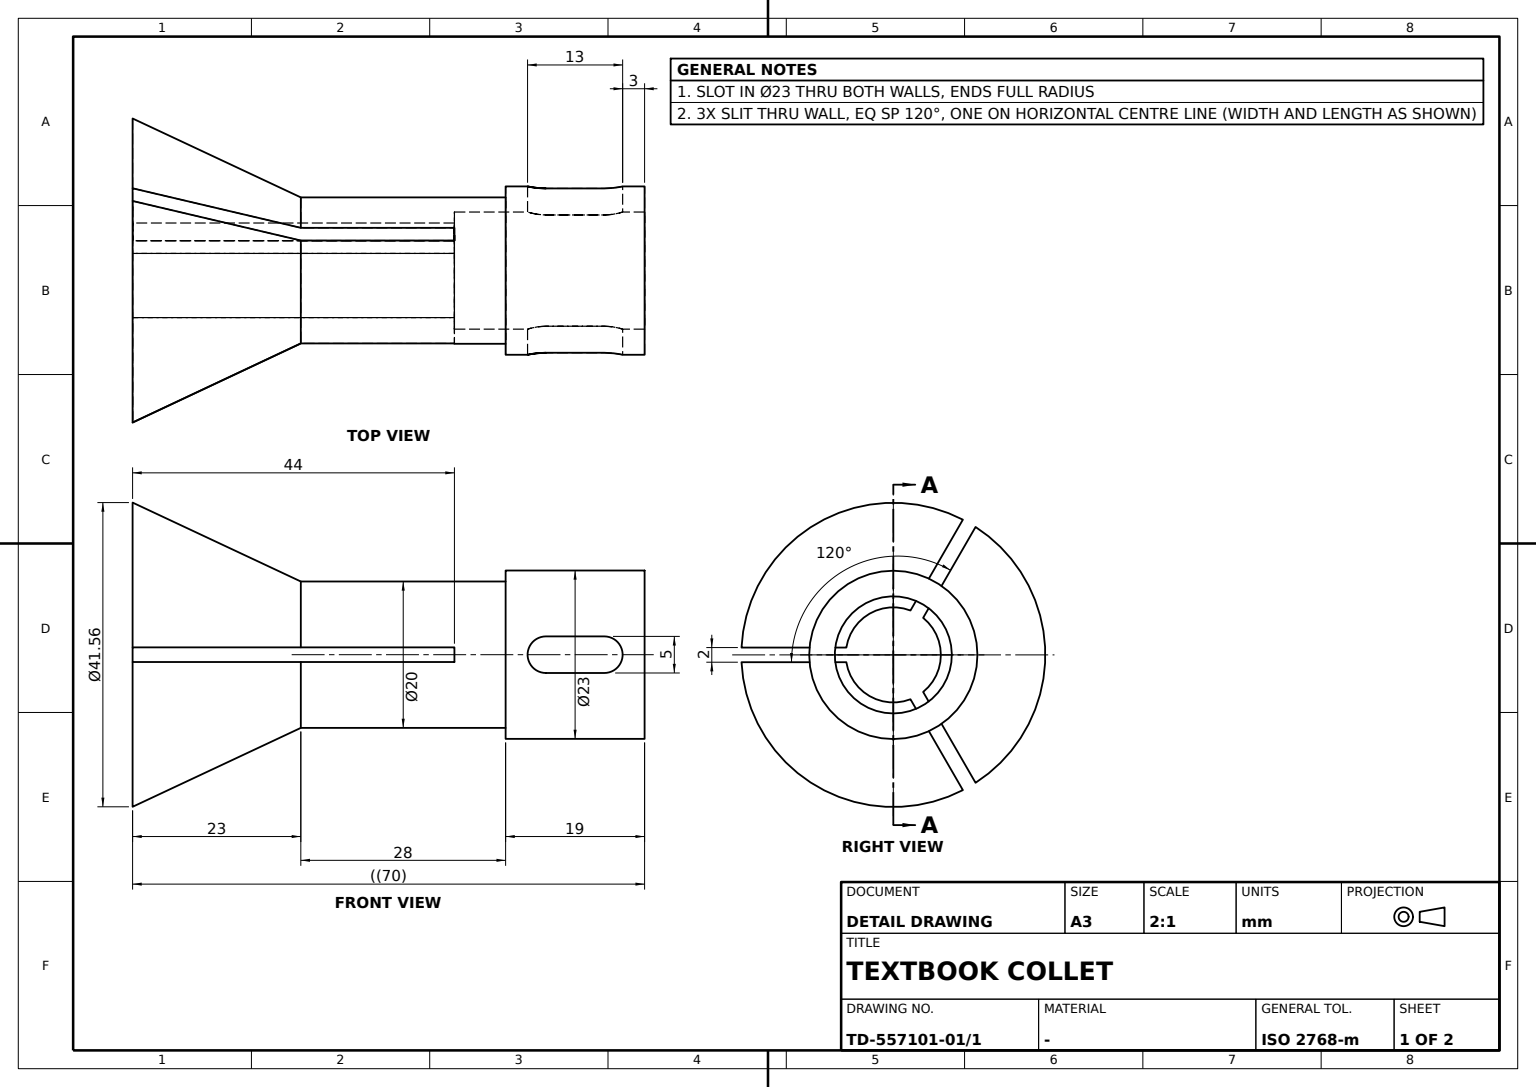
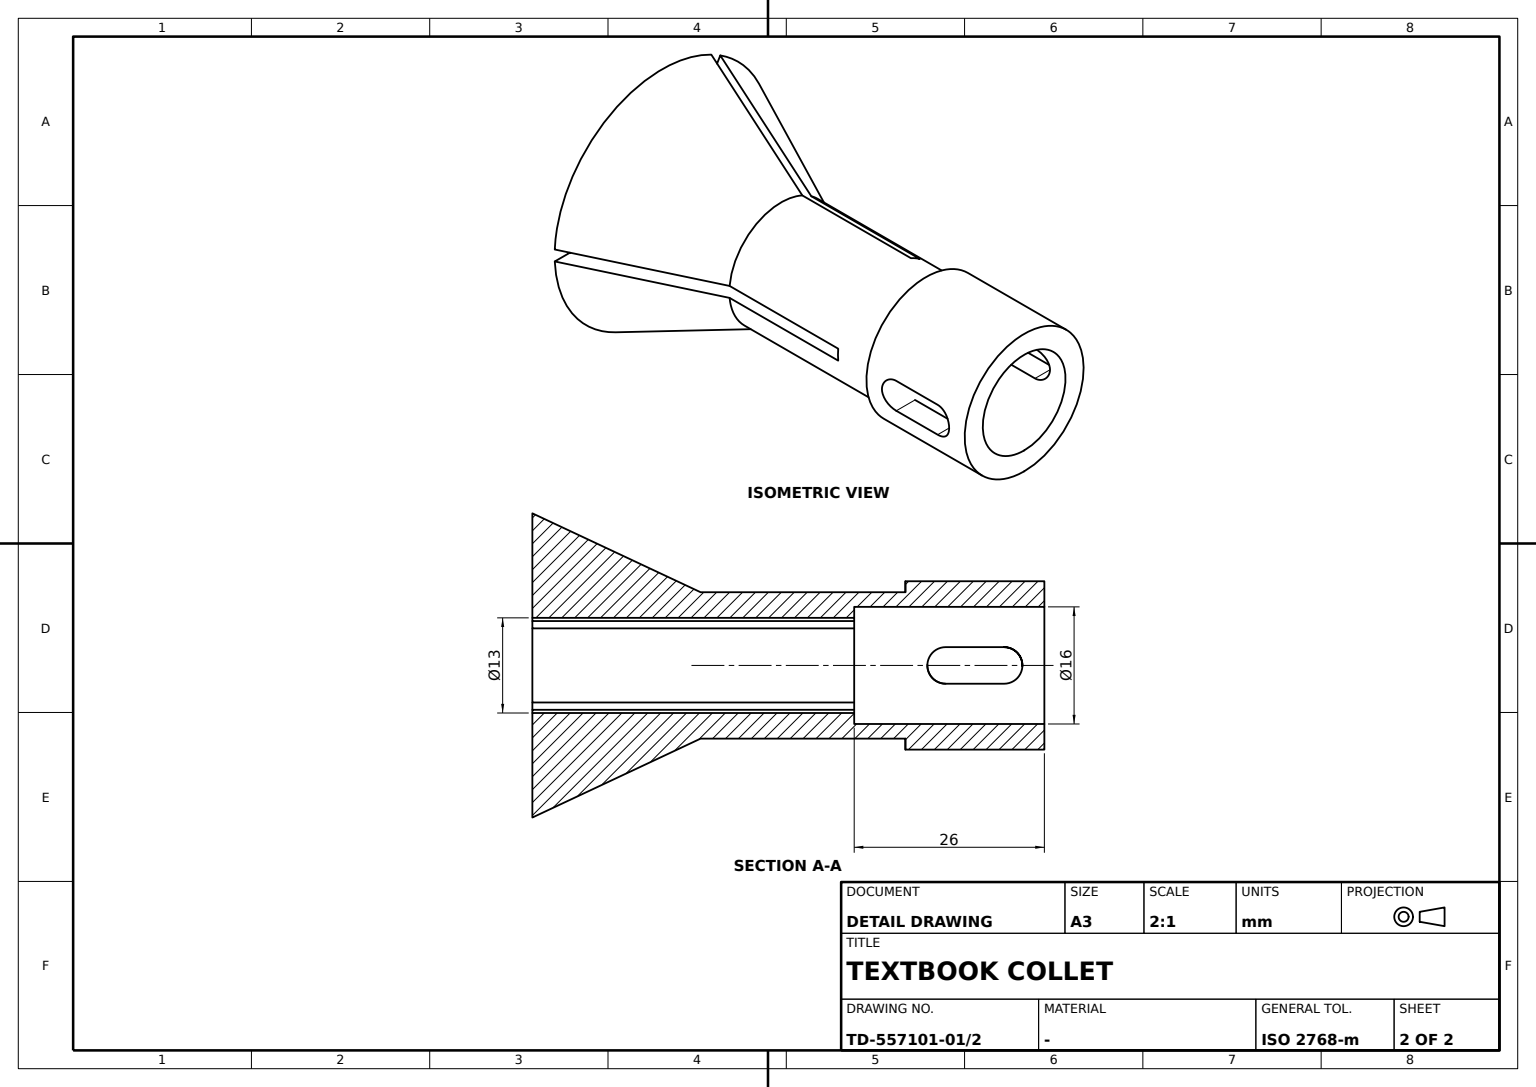
ISO-10303-21;
HEADER;
FILE_DESCRIPTION((''),'2;1');
FILE_NAME('','',(''),(''),'','','');
FILE_SCHEMA(('AUTOMOTIVE_DESIGN'));
ENDSEC;
DATA;
#1=APPLICATION_CONTEXT('');
#2=PRODUCT_CONTEXT('',#1,'mechanical');
#3=PRODUCT('','','',(#2));
#4=PRODUCT_DEFINITION_FORMATION('','',#3);
#5=PRODUCT_DEFINITION_CONTEXT('',#1,'design');
#6=PRODUCT_DEFINITION('','',#4,#5);
#7=PRODUCT_DEFINITION_SHAPE('','',#6);
#8=(LENGTH_UNIT()NAMED_UNIT(*)SI_UNIT(.MILLI.,.METRE.));
#9=(NAMED_UNIT(*)PLANE_ANGLE_UNIT()SI_UNIT($,.RADIAN.));
#10=(NAMED_UNIT(*)SI_UNIT($,.STERADIAN.)SOLID_ANGLE_UNIT());
#11=UNCERTAINTY_MEASURE_WITH_UNIT(LENGTH_MEASURE(0.005),#8,'distance_accuracy_value','');
#12=(GEOMETRIC_REPRESENTATION_CONTEXT(3)GLOBAL_UNCERTAINTY_ASSIGNED_CONTEXT((#11))GLOBAL_UNIT_ASSIGNED_CONTEXT((#8,#9,#10))REPRESENTATION_CONTEXT('',''));
#13=CARTESIAN_POINT('',(-47.,-9.949874,-1.));
#14=VERTEX_POINT('',#13);
#15=CARTESIAN_POINT('',(-47.,4.108912,-9.116844));
#16=VERTEX_POINT('',#15);
#17=CARTESIAN_POINT('',(-47.,0.,0.));
#18=DIRECTION('',(-1.,0.,0.));
#19=DIRECTION('',(0.,0.,1.));
#20=AXIS2_PLACEMENT_3D('',#17,#18,#19);
#21=CIRCLE('',#20,10.);
#22=EDGE_CURVE('',#14,#16,#21,.F.);
#23=ORIENTED_EDGE('',*,*,#22,.T.);
#24=CARTESIAN_POINT('',(-26.,4.108912,-9.116844));
#25=VERTEX_POINT('',#24);
#26=DIRECTION('',(1.,0.,0.));
#27=VECTOR('',#26,1000.);
#28=LINE('',#24,#27);
#29=EDGE_CURVE('',#25,#16,#28,.F.);
#30=ORIENTED_EDGE('',*,*,#29,.F.);
#31=CARTESIAN_POINT('',(-26.,5.840963,-8.116844));
#32=VERTEX_POINT('',#31);
#33=CARTESIAN_POINT('',(-26.,0.,0.));
#34=AXIS2_PLACEMENT_3D('',#33,#18,#19);
#35=CIRCLE('',#34,10.);
#36=EDGE_CURVE('',#32,#25,#35,.T.);
#37=ORIENTED_EDGE('',*,*,#36,.F.);
#38=CARTESIAN_POINT('',(-47.,5.840963,-8.116844));
#39=VERTEX_POINT('',#38);
#40=LINE('',#31,#27);
#41=EDGE_CURVE('',#32,#39,#40,.F.);
#42=ORIENTED_EDGE('',*,*,#41,.T.);
#43=CARTESIAN_POINT('',(-47.,5.840963,8.116844));
#44=VERTEX_POINT('',#43);
#45=EDGE_CURVE('',#39,#44,#21,.F.);
#46=ORIENTED_EDGE('',*,*,#45,.T.);
#47=CARTESIAN_POINT('',(-26.,5.840963,8.116844));
#48=VERTEX_POINT('',#47);
#49=LINE('',#47,#27);
#50=EDGE_CURVE('',#48,#44,#49,.F.);
#51=ORIENTED_EDGE('',*,*,#50,.F.);
#52=CARTESIAN_POINT('',(-26.,4.108912,9.116844));
#53=VERTEX_POINT('',#52);
#54=EDGE_CURVE('',#53,#48,#35,.T.);
#55=ORIENTED_EDGE('',*,*,#54,.F.);
#56=CARTESIAN_POINT('',(-47.,4.108912,9.116844));
#57=VERTEX_POINT('',#56);
#58=LINE('',#52,#27);
#59=EDGE_CURVE('',#53,#57,#58,.F.);
#60=ORIENTED_EDGE('',*,*,#59,.T.);
#61=CARTESIAN_POINT('',(-47.,-9.949874,1.));
#62=VERTEX_POINT('',#61);
#63=EDGE_CURVE('',#57,#62,#21,.F.);
#64=ORIENTED_EDGE('',*,*,#63,.T.);
#65=CARTESIAN_POINT('',(-26.,-9.949874,1.));
#66=VERTEX_POINT('',#65);
#67=LINE('',#61,#27);
#68=EDGE_CURVE('',#62,#66,#67,.T.);
#69=ORIENTED_EDGE('',*,*,#68,.T.);
#70=CARTESIAN_POINT('',(-26.,-9.949874,-1.));
#71=VERTEX_POINT('',#70);
#72=EDGE_CURVE('',#71,#66,#35,.T.);
#73=ORIENTED_EDGE('',*,*,#72,.F.);
#74=LINE('',#13,#27);
#75=EDGE_CURVE('',#14,#71,#74,.T.);
#76=ORIENTED_EDGE('',*,*,#75,.F.);
#77=EDGE_LOOP('',(#23,#30,#37,#42,#46,#51,#55,#60,#64,#69,#73,#76));
#78=FACE_BOUND('',#77,.T.);
#79=CARTESIAN_POINT('',(-19.,0.,-10.));
#80=VERTEX_POINT('',#79);
#81=CARTESIAN_POINT('',(-19.,0.,0.));
#82=DIRECTION('',(0.,0.,-1.));
#83=AXIS2_PLACEMENT_3D('',#81,#26,#82);
#84=CIRCLE('',#83,10.);
#85=EDGE_CURVE('',#80,#80,#84,.T.);
#86=ORIENTED_EDGE('',*,*,#85,.F.);
#87=EDGE_LOOP('',(#86));
#88=FACE_BOUND('',#87,.T.);
#89=CARTESIAN_POINT('',(-35.,0.,0.));
#90=DIRECTION('',(0.,1.,0.));
#91=AXIS2_PLACEMENT_3D('',#89,#26,#90);
#92=CYLINDRICAL_SURFACE('',#91,10.);
#93=ADVANCED_FACE('',(#78,#88),#92,.T.);
#94=CARTESIAN_POINT('',(-70.,9.511937,18.475158));
#95=VERTEX_POINT('',#94);
#96=CARTESIAN_POINT('',(-54.663041,5.913776,12.24296));
#97=CARTESIAN_POINT('',(-62.331595,7.712778,15.358924));
#98=B_SPLINE_CURVE_WITH_KNOTS('',3,(#56,#96,#97,#94),.UNSPECIFIED.,.F.,.F.,(4,4),(0.,0.025412019),.UNSPECIFIED.);
#99=EDGE_CURVE('',#57,#95,#98,.T.);
#100=ORIENTED_EDGE('',*,*,#99,.F.);
#101=ORIENTED_EDGE('',*,*,#59,.F.);
#102=CARTESIAN_POINT('',(-26.,3.102602,7.373864));
#103=VERTEX_POINT('',#102);
#104=CARTESIAN_POINT('',(-26.,9.511937,18.475158));
#105=DIRECTION('',(0.,-0.5,-0.866025404));
#106=VECTOR('',#105,1000.);
#107=LINE('',#104,#106);
#108=EDGE_CURVE('',#53,#103,#107,.T.);
#109=ORIENTED_EDGE('',*,*,#108,.T.);
#110=CARTESIAN_POINT('',(-26.,2.345283,6.062149));
#111=VERTEX_POINT('',#110);
#112=EDGE_CURVE('',#103,#111,#107,.T.);
#113=ORIENTED_EDGE('',*,*,#112,.T.);
#114=CARTESIAN_POINT('',(-70.,2.345283,6.062149));
#115=VERTEX_POINT('',#114);
#116=VECTOR('',#18,1000.);
#117=LINE('',#114,#116);
#118=EDGE_CURVE('',#115,#111,#117,.F.);
#119=ORIENTED_EDGE('',*,*,#118,.F.);
#120=CARTESIAN_POINT('',(-70.,8.131979,16.085));
#121=LINE('',#120,#106);
#122=EDGE_CURVE('',#95,#115,#121,.T.);
#123=ORIENTED_EDGE('',*,*,#122,.F.);
#124=EDGE_LOOP('',(#100,#101,#109,#113,#119,#123));
#125=FACE_BOUND('',#124,.T.);
#126=DIRECTION('',(0.,-0.866025404,0.5));
#127=AXIS2_PLACEMENT_3D('',#94,#126,#105);
#128=PLANE('',#127);
#129=ADVANCED_FACE('',(#125),#128,.F.);
#130=CARTESIAN_POINT('',(-13.5,-11.224972,2.5));
#131=VERTEX_POINT('',#130);
#132=CARTESIAN_POINT('',(-13.5,-7.599342,2.5));
#133=VERTEX_POINT('',#132);
#134=CARTESIAN_POINT('',(-13.5,5.3,2.5));
#135=VECTOR('',#90,1000.);
#136=LINE('',#134,#135);
#137=EDGE_CURVE('',#131,#133,#136,.T.);
#138=ORIENTED_EDGE('',*,*,#137,.T.);
#139=CARTESIAN_POINT('',(-5.5,-7.599342,2.5));
#140=VERTEX_POINT('',#139);
#141=LINE('',#139,#27);
#142=EDGE_CURVE('',#133,#140,#141,.T.);
#143=ORIENTED_EDGE('',*,*,#142,.T.);
#144=CARTESIAN_POINT('',(-5.5,-11.224972,2.5));
#145=VERTEX_POINT('',#144);
#146=CARTESIAN_POINT('',(-5.5,5.3,2.5));
#147=LINE('',#146,#135);
#148=EDGE_CURVE('',#145,#140,#147,.T.);
#149=ORIENTED_EDGE('',*,*,#148,.F.);
#150=LINE('',#144,#27);
#151=EDGE_CURVE('',#145,#131,#150,.F.);
#152=ORIENTED_EDGE('',*,*,#151,.T.);
#153=EDGE_LOOP('',(#138,#143,#149,#152));
#154=FACE_BOUND('',#153,.T.);
#155=CARTESIAN_POINT('',(-5.5,-11.5,2.5));
#156=AXIS2_PLACEMENT_3D('',#155,#82,#18);
#157=PLANE('',#156);
#158=ADVANCED_FACE('',(#154),#157,.T.);
#159=CARTESIAN_POINT('',(-70.,9.511937,-18.475158));
#160=VERTEX_POINT('',#159);
#161=CARTESIAN_POINT('',(-54.663041,5.913776,-12.24296));
#162=CARTESIAN_POINT('',(-62.331595,7.712778,-15.358924));
#163=B_SPLINE_CURVE_WITH_KNOTS('',3,(#15,#161,#162,#159),.UNSPECIFIED.,.F.,.F.,(4,4),(0.,0.025412019),.UNSPECIFIED.);
#164=EDGE_CURVE('',#16,#160,#163,.T.);
#165=ORIENTED_EDGE('',*,*,#164,.T.);
#166=CARTESIAN_POINT('',(-70.,2.345283,-6.062149));
#167=VERTEX_POINT('',#166);
#168=CARTESIAN_POINT('',(-70.,-9.864029,15.085));
#169=DIRECTION('',(0.,0.5,-0.866025404));
#170=VECTOR('',#169,1000.);
#171=LINE('',#168,#170);
#172=EDGE_CURVE('',#167,#160,#171,.T.);
#173=ORIENTED_EDGE('',*,*,#172,.F.);
#174=CARTESIAN_POINT('',(-26.,2.345283,-6.062149));
#175=VERTEX_POINT('',#174);
#176=LINE('',#166,#116);
#177=EDGE_CURVE('',#167,#175,#176,.F.);
#178=ORIENTED_EDGE('',*,*,#177,.T.);
#179=CARTESIAN_POINT('',(-26.,3.102602,-7.373864));
#180=VERTEX_POINT('',#179);
#181=LINE('',#174,#170);
#182=EDGE_CURVE('',#175,#180,#181,.T.);
#183=ORIENTED_EDGE('',*,*,#182,.T.);
#184=EDGE_CURVE('',#180,#25,#181,.T.);
#185=ORIENTED_EDGE('',*,*,#184,.T.);
#186=ORIENTED_EDGE('',*,*,#29,.T.);
#187=EDGE_LOOP('',(#165,#173,#178,#183,#185,#186));
#188=FACE_BOUND('',#187,.T.);
#189=DIRECTION('',(0.,-0.866025404,-0.5));
#190=AXIS2_PLACEMENT_3D('',#166,#189,#169);
#191=PLANE('',#190);
#192=ADVANCED_FACE('',(#188),#191,.F.);
#193=ORIENTED_EDGE('',*,*,#118,.T.);
#194=CARTESIAN_POINT('',(-26.,-6.422616,1.));
#195=VERTEX_POINT('',#194);
#196=CIRCLE('',#34,6.5);
#197=EDGE_CURVE('',#195,#111,#196,.T.);
#198=ORIENTED_EDGE('',*,*,#197,.F.);
#199=CARTESIAN_POINT('',(-70.,-6.422616,1.));
#200=VERTEX_POINT('',#199);
#201=LINE('',#199,#116);
#202=EDGE_CURVE('',#200,#195,#201,.F.);
#203=ORIENTED_EDGE('',*,*,#202,.F.);
#204=CARTESIAN_POINT('',(-70.,0.,0.));
#205=AXIS2_PLACEMENT_3D('',#204,#26,#82);
#206=CIRCLE('',#205,6.5);
#207=EDGE_CURVE('',#200,#115,#206,.F.);
#208=ORIENTED_EDGE('',*,*,#207,.T.);
#209=EDGE_LOOP('',(#193,#198,#203,#208));
#210=FACE_BOUND('',#209,.T.);
#211=CARTESIAN_POINT('',(-48.,0.,0.));
#212=DIRECTION('',(0.,-1.,0.));
#213=AXIS2_PLACEMENT_3D('',#211,#18,#212);
#214=CYLINDRICAL_SURFACE('',#213,6.5);
#215=ADVANCED_FACE('',(#210),#214,.F.);
#216=ORIENTED_EDGE('',*,*,#36,.T.);
#217=ORIENTED_EDGE('',*,*,#184,.F.);
#218=CARTESIAN_POINT('',(-26.,4.834652,-6.373864));
#219=VERTEX_POINT('',#218);
#220=CIRCLE('',#34,8.);
#221=EDGE_CURVE('',#180,#219,#220,.F.);
#222=ORIENTED_EDGE('',*,*,#221,.T.);
#223=CARTESIAN_POINT('',(-26.,11.243988,-17.475158));
#224=DIRECTION('',(0.,-0.5,0.866025404));
#225=VECTOR('',#224,1000.);
#226=LINE('',#223,#225);
#227=EDGE_CURVE('',#32,#219,#226,.T.);
#228=ORIENTED_EDGE('',*,*,#227,.F.);
#229=EDGE_LOOP('',(#216,#217,#222,#228));
#230=FACE_BOUND('',#229,.T.);
#231=AXIS2_PLACEMENT_3D('',#33,#18,#212);
#232=PLANE('',#231);
#233=ADVANCED_FACE('',(#230),#232,.T.);
#234=CARTESIAN_POINT('',(-70.,4.077334,5.062149));
#235=VERTEX_POINT('',#234);
#236=CARTESIAN_POINT('',(-70.,11.243988,17.475158));
#237=VERTEX_POINT('',#236);
#238=CARTESIAN_POINT('',(-70.,9.864029,15.085));
#239=DIRECTION('',(0.,0.5,0.866025404));
#240=VECTOR('',#239,1000.);
#241=LINE('',#238,#240);
#242=EDGE_CURVE('',#235,#237,#241,.T.);
#243=ORIENTED_EDGE('',*,*,#242,.T.);
#244=CARTESIAN_POINT('',(-70.,11.243988,-17.475158));
#245=VERTEX_POINT('',#244);
#246=CIRCLE('',#205,20.78);
#247=EDGE_CURVE('',#245,#237,#246,.T.);
#248=ORIENTED_EDGE('',*,*,#247,.F.);
#249=CARTESIAN_POINT('',(-70.,4.077334,-5.062149));
#250=VERTEX_POINT('',#249);
#251=CARTESIAN_POINT('',(-70.,-8.131979,16.085));
#252=LINE('',#251,#225);
#253=EDGE_CURVE('',#245,#250,#252,.T.);
#254=ORIENTED_EDGE('',*,*,#253,.T.);
#255=EDGE_CURVE('',#235,#250,#206,.F.);
#256=ORIENTED_EDGE('',*,*,#255,.F.);
#257=EDGE_LOOP('',(#243,#248,#254,#256));
#258=FACE_BOUND('',#257,.T.);
#259=CARTESIAN_POINT('',(-70.,0.,20.78));
#260=AXIS2_PLACEMENT_3D('',#259,#26,#90);
#261=PLANE('',#260);
#262=ADVANCED_FACE('',(#258),#261,.F.);
#263=CARTESIAN_POINT('',(-26.,-7.937254,-1.));
#264=VERTEX_POINT('',#263);
#265=CARTESIAN_POINT('',(-26.,-6.422616,-1.));
#266=VERTEX_POINT('',#265);
#267=CARTESIAN_POINT('',(-26.,-20.755924,-1.));
#268=LINE('',#267,#135);
#269=EDGE_CURVE('',#264,#266,#268,.T.);
#270=ORIENTED_EDGE('',*,*,#269,.F.);
#271=EDGE_CURVE('',#264,#180,#220,.F.);
#272=ORIENTED_EDGE('',*,*,#271,.T.);
#273=ORIENTED_EDGE('',*,*,#182,.F.);
#274=EDGE_CURVE('',#175,#266,#196,.T.);
#275=ORIENTED_EDGE('',*,*,#274,.T.);
#276=EDGE_LOOP('',(#270,#272,#273,#275));
#277=FACE_BOUND('',#276,.T.);
#278=ADVANCED_FACE('',(#277),#232,.F.);
#279=CARTESIAN_POINT('',(-70.,-20.755924,-1.));
#280=VERTEX_POINT('',#279);
#281=CARTESIAN_POINT('',(-70.,-6.422616,-1.));
#282=VERTEX_POINT('',#281);
#283=CARTESIAN_POINT('',(-70.,0.,-1.));
#284=LINE('',#283,#135);
#285=EDGE_CURVE('',#280,#282,#284,.T.);
#286=ORIENTED_EDGE('',*,*,#285,.F.);
#287=CARTESIAN_POINT('',(-54.663041,-13.559603,-1.));
#288=CARTESIAN_POINT('',(-62.331595,-17.157607,-1.));
#289=B_SPLINE_CURVE_WITH_KNOTS('',3,(#13,#287,#288,#279),.UNSPECIFIED.,.F.,.F.,(4,4),(0.,0.025412019),.UNSPECIFIED.);
#290=EDGE_CURVE('',#14,#280,#289,.T.);
#291=ORIENTED_EDGE('',*,*,#290,.F.);
#292=ORIENTED_EDGE('',*,*,#75,.T.);
#293=EDGE_CURVE('',#71,#264,#268,.T.);
#294=ORIENTED_EDGE('',*,*,#293,.T.);
#295=ORIENTED_EDGE('',*,*,#269,.T.);
#296=LINE('',#281,#116);
#297=EDGE_CURVE('',#282,#266,#296,.F.);
#298=ORIENTED_EDGE('',*,*,#297,.F.);
#299=EDGE_LOOP('',(#286,#291,#292,#294,#295,#298));
#300=FACE_BOUND('',#299,.T.);
#301=AXIS2_PLACEMENT_3D('',#279,#82,#90);
#302=PLANE('',#301);
#303=ADVANCED_FACE('',(#300),#302,.F.);
#304=ORIENTED_EDGE('',*,*,#85,.T.);
#305=EDGE_LOOP('',(#304));
#306=FACE_BOUND('',#305,.T.);
#307=CARTESIAN_POINT('',(-19.,0.,-11.5));
#308=VERTEX_POINT('',#307);
#309=CIRCLE('',#83,11.5);
#310=EDGE_CURVE('',#308,#308,#309,.T.);
#311=ORIENTED_EDGE('',*,*,#310,.F.);
#312=EDGE_LOOP('',(#311));
#313=FACE_BOUND('',#312,.T.);
#314=CARTESIAN_POINT('',(-19.,0.,11.5));
#315=AXIS2_PLACEMENT_3D('',#314,#26,#90);
#316=PLANE('',#315);
#317=ADVANCED_FACE('',(#306,#313),#316,.F.);
#318=CARTESIAN_POINT('',(-26.,-7.937254,1.));
#319=VERTEX_POINT('',#318);
#320=VECTOR('',#212,1000.);
#321=LINE('',#194,#320);
#322=EDGE_CURVE('',#319,#66,#321,.T.);
#323=ORIENTED_EDGE('',*,*,#322,.F.);
#324=EDGE_CURVE('',#319,#264,#220,.F.);
#325=ORIENTED_EDGE('',*,*,#324,.T.);
#326=ORIENTED_EDGE('',*,*,#293,.F.);
#327=ORIENTED_EDGE('',*,*,#72,.T.);
#328=EDGE_LOOP('',(#323,#325,#326,#327));
#329=FACE_BOUND('',#328,.T.);
#330=ADVANCED_FACE('',(#329),#232,.T.);
#331=ORIENTED_EDGE('',*,*,#54,.T.);
#332=CARTESIAN_POINT('',(-26.,4.834652,6.373864));
#333=VERTEX_POINT('',#332);
#334=CARTESIAN_POINT('',(-26.,4.077334,5.062149));
#335=LINE('',#334,#240);
#336=EDGE_CURVE('',#333,#48,#335,.T.);
#337=ORIENTED_EDGE('',*,*,#336,.F.);
#338=EDGE_CURVE('',#333,#103,#220,.F.);
#339=ORIENTED_EDGE('',*,*,#338,.T.);
#340=ORIENTED_EDGE('',*,*,#108,.F.);
#341=EDGE_LOOP('',(#331,#337,#339,#340));
#342=FACE_BOUND('',#341,.T.);
#343=ADVANCED_FACE('',(#342),#232,.T.);
#344=VERTEX_POINT('',#334);
#345=LINE('',#234,#116);
#346=EDGE_CURVE('',#235,#344,#345,.F.);
#347=ORIENTED_EDGE('',*,*,#346,.F.);
#348=ORIENTED_EDGE('',*,*,#255,.T.);
#349=CARTESIAN_POINT('',(-26.,4.077334,-5.062149));
#350=VERTEX_POINT('',#349);
#351=LINE('',#249,#116);
#352=EDGE_CURVE('',#250,#350,#351,.F.);
#353=ORIENTED_EDGE('',*,*,#352,.T.);
#354=EDGE_CURVE('',#344,#350,#196,.T.);
#355=ORIENTED_EDGE('',*,*,#354,.F.);
#356=EDGE_LOOP('',(#347,#348,#353,#355));
#357=FACE_BOUND('',#356,.T.);
#358=ADVANCED_FACE('',(#357),#214,.F.);
#359=ORIENTED_EDGE('',*,*,#336,.T.);
#360=ORIENTED_EDGE('',*,*,#50,.T.);
#361=CARTESIAN_POINT('',(-54.663041,7.645827,11.24296));
#362=CARTESIAN_POINT('',(-62.331595,9.444829,14.358924));
#363=B_SPLINE_CURVE_WITH_KNOTS('',3,(#43,#361,#362,#236),.UNSPECIFIED.,.F.,.F.,(4,4),(0.,0.025412019),.UNSPECIFIED.);
#364=EDGE_CURVE('',#44,#237,#363,.T.);
#365=ORIENTED_EDGE('',*,*,#364,.T.);
#366=ORIENTED_EDGE('',*,*,#242,.F.);
#367=ORIENTED_EDGE('',*,*,#346,.T.);
#368=EDGE_CURVE('',#344,#333,#335,.T.);
#369=ORIENTED_EDGE('',*,*,#368,.T.);
#370=EDGE_LOOP('',(#359,#360,#365,#366,#367,#369));
#371=FACE_BOUND('',#370,.T.);
#372=DIRECTION('',(0.,0.866025404,-0.5));
#373=AXIS2_PLACEMENT_3D('',#234,#372,#239);
#374=PLANE('',#373);
#375=ADVANCED_FACE('',(#371),#374,.F.);
#376=CARTESIAN_POINT('',(-5.5,-7.599342,-2.5));
#377=VERTEX_POINT('',#376);
#378=CARTESIAN_POINT('',(-13.5,-7.599342,-2.5));
#379=VERTEX_POINT('',#378);
#380=LINE('',#378,#27);
#381=EDGE_CURVE('',#377,#379,#380,.F.);
#382=ORIENTED_EDGE('',*,*,#381,.T.);
#383=CARTESIAN_POINT('',(-13.5,-11.224972,-2.5));
#384=VERTEX_POINT('',#383);
#385=CARTESIAN_POINT('',(-13.5,5.3,-2.5));
#386=LINE('',#385,#135);
#387=EDGE_CURVE('',#384,#379,#386,.T.);
#388=ORIENTED_EDGE('',*,*,#387,.F.);
#389=CARTESIAN_POINT('',(-5.5,-11.224972,-2.5));
#390=VERTEX_POINT('',#389);
#391=LINE('',#383,#27);
#392=EDGE_CURVE('',#384,#390,#391,.T.);
#393=ORIENTED_EDGE('',*,*,#392,.T.);
#394=CARTESIAN_POINT('',(-5.5,5.3,-2.5));
#395=LINE('',#394,#135);
#396=EDGE_CURVE('',#390,#377,#395,.T.);
#397=ORIENTED_EDGE('',*,*,#396,.T.);
#398=EDGE_LOOP('',(#382,#388,#393,#397));
#399=FACE_BOUND('',#398,.T.);
#400=CARTESIAN_POINT('',(-13.5,-11.5,-2.5));
#401=AXIS2_PLACEMENT_3D('',#400,#19,#26);
#402=PLANE('',#401);
#403=ADVANCED_FACE('',(#399),#402,.T.);
#404=CARTESIAN_POINT('',(-5.5,7.599342,2.5));
#405=VERTEX_POINT('',#404);
#406=CARTESIAN_POINT('',(-5.5,11.224972,2.5));
#407=VERTEX_POINT('',#406);
#408=EDGE_CURVE('',#405,#407,#147,.T.);
#409=ORIENTED_EDGE('',*,*,#408,.F.);
#410=CARTESIAN_POINT('',(-13.5,7.599342,2.5));
#411=VERTEX_POINT('',#410);
#412=LINE('',#404,#27);
#413=EDGE_CURVE('',#405,#411,#412,.F.);
#414=ORIENTED_EDGE('',*,*,#413,.T.);
#415=CARTESIAN_POINT('',(-13.5,11.224972,2.5));
#416=VERTEX_POINT('',#415);
#417=EDGE_CURVE('',#411,#416,#136,.T.);
#418=ORIENTED_EDGE('',*,*,#417,.T.);
#419=LINE('',#406,#27);
#420=EDGE_CURVE('',#416,#407,#419,.T.);
#421=ORIENTED_EDGE('',*,*,#420,.T.);
#422=EDGE_LOOP('',(#409,#414,#418,#421));
#423=FACE_BOUND('',#422,.T.);
#424=ADVANCED_FACE('',(#423),#157,.T.);
#425=EDGE_CURVE('',#219,#350,#226,.T.);
#426=ORIENTED_EDGE('',*,*,#425,.F.);
#427=EDGE_CURVE('',#219,#333,#220,.F.);
#428=ORIENTED_EDGE('',*,*,#427,.T.);
#429=ORIENTED_EDGE('',*,*,#368,.F.);
#430=ORIENTED_EDGE('',*,*,#354,.T.);
#431=EDGE_LOOP('',(#426,#428,#429,#430));
#432=FACE_BOUND('',#431,.T.);
#433=ADVANCED_FACE('',(#432),#232,.F.);
#434=EDGE_CURVE('',#280,#160,#246,.T.);
#435=ORIENTED_EDGE('',*,*,#434,.F.);
#436=ORIENTED_EDGE('',*,*,#285,.T.);
#437=EDGE_CURVE('',#167,#282,#206,.F.);
#438=ORIENTED_EDGE('',*,*,#437,.F.);
#439=ORIENTED_EDGE('',*,*,#172,.T.);
#440=EDGE_LOOP('',(#435,#436,#438,#439));
#441=FACE_BOUND('',#440,.T.);
#442=ADVANCED_FACE('',(#441),#261,.F.);
#443=CARTESIAN_POINT('',(-13.5,7.599342,-2.5));
#444=VERTEX_POINT('',#443);
#445=CARTESIAN_POINT('',(-13.5,11.224972,-2.5));
#446=VERTEX_POINT('',#445);
#447=EDGE_CURVE('',#444,#446,#386,.T.);
#448=ORIENTED_EDGE('',*,*,#447,.T.);
#449=CARTESIAN_POINT('',(-14.162676,11.224972,-2.5));
#450=CARTESIAN_POINT('',(-15.454326,11.364171,-1.9581));
#451=CARTESIAN_POINT('',(-16.272468,11.567857,-0.00323));
#452=CARTESIAN_POINT('',(-15.455797,11.3644,1.958471));
#453=CARTESIAN_POINT('',(-14.162684,11.224972,2.5));
#454=B_SPLINE_CURVE_WITH_KNOTS('',3,(#445,#449,#450,#451,#452,#453,#415),.UNSPECIFIED.,.F.,.F.,(4,1,1,1,4),(0.,0.001959339,0.003918677,0.005878016,0.007837355),.UNSPECIFIED.);
#455=EDGE_CURVE('',#446,#416,#454,.T.);
#456=ORIENTED_EDGE('',*,*,#455,.T.);
#457=ORIENTED_EDGE('',*,*,#417,.F.);
#458=CARTESIAN_POINT('',(-14.165012,7.599342,-2.5));
#459=CARTESIAN_POINT('',(-15.452827,7.80477,-1.958108));
#460=CARTESIAN_POINT('',(-16.273308,8.09755,-0.004106));
#461=CARTESIAN_POINT('',(-15.453934,7.805026,1.959324));
#462=CARTESIAN_POINT('',(-14.165065,7.599342,2.5));
#463=B_SPLINE_CURVE_WITH_KNOTS('',3,(#443,#458,#459,#460,#461,#462,#410),.UNSPECIFIED.,.F.,.F.,(4,1,1,1,4),(0.,0.001965679,0.003931357,0.005897036,0.007862715),.UNSPECIFIED.);
#464=EDGE_CURVE('',#444,#411,#463,.T.);
#465=ORIENTED_EDGE('',*,*,#464,.F.);
#466=EDGE_LOOP('',(#448,#456,#457,#465));
#467=FACE_BOUND('',#466,.T.);
#468=CARTESIAN_POINT('',(-13.5,5.3,0.));
#469=AXIS2_PLACEMENT_3D('',#468,#90,#19);
#470=CYLINDRICAL_SURFACE('',#469,2.5);
#471=ADVANCED_FACE('',(#467),#470,.F.);
#472=ORIENTED_EDGE('',*,*,#197,.T.);
#473=ORIENTED_EDGE('',*,*,#112,.F.);
#474=EDGE_CURVE('',#103,#319,#220,.F.);
#475=ORIENTED_EDGE('',*,*,#474,.T.);
#476=EDGE_CURVE('',#195,#319,#321,.T.);
#477=ORIENTED_EDGE('',*,*,#476,.F.);
#478=EDGE_LOOP('',(#472,#473,#475,#477));
#479=FACE_BOUND('',#478,.T.);
#480=ADVANCED_FACE('',(#479),#232,.F.);
#481=CARTESIAN_POINT('',(-70.,-20.755924,1.));
#482=VERTEX_POINT('',#481);
#483=CARTESIAN_POINT('',(-54.663041,-13.559603,1.));
#484=CARTESIAN_POINT('',(-62.331595,-17.157607,1.));
#485=B_SPLINE_CURVE_WITH_KNOTS('',3,(#61,#483,#484,#481),.UNSPECIFIED.,.F.,.F.,(4,4),(0.,0.025412019),.UNSPECIFIED.);
#486=EDGE_CURVE('',#62,#482,#485,.T.);
#487=ORIENTED_EDGE('',*,*,#486,.T.);
#488=CARTESIAN_POINT('',(-70.,0.,1.));
#489=LINE('',#488,#320);
#490=EDGE_CURVE('',#200,#482,#489,.T.);
#491=ORIENTED_EDGE('',*,*,#490,.F.);
#492=ORIENTED_EDGE('',*,*,#202,.T.);
#493=ORIENTED_EDGE('',*,*,#476,.T.);
#494=ORIENTED_EDGE('',*,*,#322,.T.);
#495=ORIENTED_EDGE('',*,*,#68,.F.);
#496=EDGE_LOOP('',(#487,#491,#492,#493,#494,#495));
#497=FACE_BOUND('',#496,.T.);
#498=AXIS2_PLACEMENT_3D('',#199,#19,#212);
#499=PLANE('',#498);
#500=ADVANCED_FACE('',(#497),#499,.F.);
#501=ORIENTED_EDGE('',*,*,#45,.F.);
#502=CARTESIAN_POINT('',(-54.663041,7.645827,-11.24296));
#503=CARTESIAN_POINT('',(-62.331595,9.444829,-14.358924));
#504=B_SPLINE_CURVE_WITH_KNOTS('',3,(#38,#502,#503,#244),.UNSPECIFIED.,.F.,.F.,(4,4),(0.,0.025412019),.UNSPECIFIED.);
#505=EDGE_CURVE('',#39,#245,#504,.T.);
#506=ORIENTED_EDGE('',*,*,#505,.T.);
#507=ORIENTED_EDGE('',*,*,#247,.T.);
#508=ORIENTED_EDGE('',*,*,#364,.F.);
#509=EDGE_LOOP('',(#501,#506,#507,#508));
#510=FACE_BOUND('',#509,.T.);
#511=AXIS2_PLACEMENT_3D('',#17,#18,#90);
#512=CONICAL_SURFACE('',#511,10.,0.438292002);
#513=ADVANCED_FACE('',(#510),#512,.T.);
#514=ORIENTED_EDGE('',*,*,#387,.T.);
#515=CARTESIAN_POINT('',(-14.165012,-7.599342,-2.5));
#516=CARTESIAN_POINT('',(-15.452827,-7.80477,-1.958108));
#517=CARTESIAN_POINT('',(-16.273308,-8.09755,-0.004106));
#518=CARTESIAN_POINT('',(-15.453934,-7.805026,1.959324));
#519=CARTESIAN_POINT('',(-14.165065,-7.599342,2.5));
#520=B_SPLINE_CURVE_WITH_KNOTS('',3,(#378,#515,#516,#517,#518,#519,#132),.UNSPECIFIED.,.F.,.F.,(4,1,1,1,4),(0.,0.001965679,0.003931357,0.005897036,0.007862715),.UNSPECIFIED.);
#521=EDGE_CURVE('',#133,#379,#520,.F.);
#522=ORIENTED_EDGE('',*,*,#521,.F.);
#523=ORIENTED_EDGE('',*,*,#137,.F.);
#524=CARTESIAN_POINT('',(-14.162419,-11.224972,-2.5));
#525=CARTESIAN_POINT('',(-15.453403,-11.364007,-1.960103));
#526=CARTESIAN_POINT('',(-16.272875,-11.567931,0.000571));
#527=CARTESIAN_POINT('',(-15.455097,-11.364268,1.958096));
#528=CARTESIAN_POINT('',(-14.162386,-11.224972,2.5));
#529=B_SPLINE_CURVE_WITH_KNOTS('',3,(#383,#524,#525,#526,#527,#528,#130),.UNSPECIFIED.,.F.,.F.,(4,1,1,1,4),(0.,0.001958579,0.003917157,0.005875736,0.007834315),.UNSPECIFIED.);
#530=EDGE_CURVE('',#131,#384,#529,.F.);
#531=ORIENTED_EDGE('',*,*,#530,.T.);
#532=EDGE_LOOP('',(#514,#522,#523,#531));
#533=FACE_BOUND('',#532,.T.);
#534=ADVANCED_FACE('',(#533),#470,.F.);
#535=CARTESIAN_POINT('',(-5.5,11.224972,-2.5));
#536=VERTEX_POINT('',#535);
#537=LINE('',#445,#27);
#538=EDGE_CURVE('',#536,#446,#537,.F.);
#539=ORIENTED_EDGE('',*,*,#538,.T.);
#540=ORIENTED_EDGE('',*,*,#447,.F.);
#541=CARTESIAN_POINT('',(-5.5,7.599342,-2.5));
#542=VERTEX_POINT('',#541);
#543=LINE('',#443,#27);
#544=EDGE_CURVE('',#444,#542,#543,.T.);
#545=ORIENTED_EDGE('',*,*,#544,.T.);
#546=EDGE_CURVE('',#542,#536,#395,.T.);
#547=ORIENTED_EDGE('',*,*,#546,.T.);
#548=EDGE_LOOP('',(#539,#540,#545,#547));
#549=FACE_BOUND('',#548,.T.);
#550=ADVANCED_FACE('',(#549),#402,.T.);
#551=EDGE_CURVE('',#95,#482,#246,.T.);
#552=ORIENTED_EDGE('',*,*,#551,.T.);
#553=ORIENTED_EDGE('',*,*,#486,.F.);
#554=ORIENTED_EDGE('',*,*,#63,.F.);
#555=ORIENTED_EDGE('',*,*,#99,.T.);
#556=EDGE_LOOP('',(#552,#553,#554,#555));
#557=FACE_BOUND('',#556,.T.);
#558=ADVANCED_FACE('',(#557),#512,.T.);
#559=ORIENTED_EDGE('',*,*,#413,.F.);
#560=CARTESIAN_POINT('',(-4.834988,7.599342,2.5));
#561=CARTESIAN_POINT('',(-3.547173,7.80477,1.958108));
#562=CARTESIAN_POINT('',(-2.726692,8.09755,0.004106));
#563=CARTESIAN_POINT('',(-3.546066,7.805026,-1.959324));
#564=CARTESIAN_POINT('',(-4.834935,7.599342,-2.5));
#565=B_SPLINE_CURVE_WITH_KNOTS('',3,(#404,#560,#561,#562,#563,#564,#541),.UNSPECIFIED.,.F.,.F.,(4,1,1,1,4),(0.,0.001965679,0.003931357,0.005897036,0.007862715),.UNSPECIFIED.);
#566=EDGE_CURVE('',#542,#405,#565,.F.);
#567=ORIENTED_EDGE('',*,*,#566,.F.);
#568=ORIENTED_EDGE('',*,*,#544,.F.);
#569=ORIENTED_EDGE('',*,*,#464,.T.);
#570=EDGE_LOOP('',(#559,#567,#568,#569));
#571=FACE_BOUND('',#570,.T.);
#572=ORIENTED_EDGE('',*,*,#271,.F.);
#573=ORIENTED_EDGE('',*,*,#324,.F.);
#574=ORIENTED_EDGE('',*,*,#474,.F.);
#575=ORIENTED_EDGE('',*,*,#338,.F.);
#576=ORIENTED_EDGE('',*,*,#427,.F.);
#577=ORIENTED_EDGE('',*,*,#221,.F.);
#578=EDGE_LOOP('',(#572,#573,#574,#575,#576,#577));
#579=FACE_BOUND('',#578,.T.);
#580=ORIENTED_EDGE('',*,*,#381,.F.);
#581=CARTESIAN_POINT('',(-4.834988,-7.599342,2.5));
#582=CARTESIAN_POINT('',(-3.547173,-7.80477,1.958108));
#583=CARTESIAN_POINT('',(-2.726692,-8.09755,0.004106));
#584=CARTESIAN_POINT('',(-3.546066,-7.805026,-1.959324));
#585=CARTESIAN_POINT('',(-4.834935,-7.599342,-2.5));
#586=B_SPLINE_CURVE_WITH_KNOTS('',3,(#139,#581,#582,#583,#584,#585,#376),.UNSPECIFIED.,.F.,.F.,(4,1,1,1,4),(0.,0.001965679,0.003931357,0.005897036,0.007862715),.UNSPECIFIED.);
#587=EDGE_CURVE('',#140,#377,#586,.T.);
#588=ORIENTED_EDGE('',*,*,#587,.F.);
#589=ORIENTED_EDGE('',*,*,#142,.F.);
#590=ORIENTED_EDGE('',*,*,#521,.T.);
#591=EDGE_LOOP('',(#580,#588,#589,#590));
#592=FACE_BOUND('',#591,.T.);
#593=CARTESIAN_POINT('',(0.,0.,-8.));
#594=VERTEX_POINT('',#593);
#595=CARTESIAN_POINT('',(0.,0.,0.));
#596=AXIS2_PLACEMENT_3D('',#595,#26,#82);
#597=CIRCLE('',#596,8.);
#598=EDGE_CURVE('',#594,#594,#597,.T.);
#599=ORIENTED_EDGE('',*,*,#598,.T.);
#600=EDGE_LOOP('',(#599));
#601=FACE_BOUND('',#600,.T.);
#602=CARTESIAN_POINT('',(-13.,0.,0.));
#603=AXIS2_PLACEMENT_3D('',#602,#26,#19);
#604=CYLINDRICAL_SURFACE('',#603,8.);
#605=ADVANCED_FACE('',(#571,#579,#592,#601),#604,.F.);
#606=ORIENTED_EDGE('',*,*,#598,.F.);
#607=EDGE_LOOP('',(#606));
#608=FACE_BOUND('',#607,.T.);
#609=CARTESIAN_POINT('',(0.,0.,-11.5));
#610=VERTEX_POINT('',#609);
#611=CIRCLE('',#596,11.5);
#612=EDGE_CURVE('',#610,#610,#611,.T.);
#613=ORIENTED_EDGE('',*,*,#612,.T.);
#614=EDGE_LOOP('',(#613));
#615=FACE_BOUND('',#614,.T.);
#616=AXIS2_PLACEMENT_3D('',#595,#26,#90);
#617=PLANE('',#616);
#618=ADVANCED_FACE('',(#608,#615),#617,.T.);
#619=ORIENTED_EDGE('',*,*,#164,.F.);
#620=ORIENTED_EDGE('',*,*,#22,.F.);
#621=ORIENTED_EDGE('',*,*,#290,.T.);
#622=ORIENTED_EDGE('',*,*,#434,.T.);
#623=EDGE_LOOP('',(#619,#620,#621,#622));
#624=FACE_BOUND('',#623,.T.);
#625=ADVANCED_FACE('',(#624),#512,.T.);
#626=ORIENTED_EDGE('',*,*,#148,.T.);
#627=ORIENTED_EDGE('',*,*,#587,.T.);
#628=ORIENTED_EDGE('',*,*,#396,.F.);
#629=CARTESIAN_POINT('',(-4.837581,-11.224972,2.5));
#630=CARTESIAN_POINT('',(-3.546597,-11.364007,1.960103));
#631=CARTESIAN_POINT('',(-2.727125,-11.567931,-0.000571));
#632=CARTESIAN_POINT('',(-3.544903,-11.364268,-1.958096));
#633=CARTESIAN_POINT('',(-4.837614,-11.224972,-2.5));
#634=B_SPLINE_CURVE_WITH_KNOTS('',3,(#144,#629,#630,#631,#632,#633,#389),.UNSPECIFIED.,.F.,.F.,(4,1,1,1,4),(-0.003917042,-0.001958498,0.000000046,0.00195859,0.003917134),.UNSPECIFIED.);
#635=EDGE_CURVE('',#145,#390,#634,.T.);
#636=ORIENTED_EDGE('',*,*,#635,.F.);
#637=EDGE_LOOP('',(#626,#627,#628,#636));
#638=FACE_BOUND('',#637,.T.);
#639=CARTESIAN_POINT('',(-5.5,5.3,0.));
#640=AXIS2_PLACEMENT_3D('',#639,#90,#19);
#641=CYLINDRICAL_SURFACE('',#640,2.5);
#642=ADVANCED_FACE('',(#638),#641,.F.);
#643=ORIENTED_EDGE('',*,*,#490,.T.);
#644=ORIENTED_EDGE('',*,*,#551,.F.);
#645=ORIENTED_EDGE('',*,*,#122,.T.);
#646=ORIENTED_EDGE('',*,*,#207,.F.);
#647=EDGE_LOOP('',(#643,#644,#645,#646));
#648=FACE_BOUND('',#647,.T.);
#649=ADVANCED_FACE('',(#648),#261,.F.);
#650=ORIENTED_EDGE('',*,*,#227,.T.);
#651=ORIENTED_EDGE('',*,*,#425,.T.);
#652=ORIENTED_EDGE('',*,*,#352,.F.);
#653=ORIENTED_EDGE('',*,*,#253,.F.);
#654=ORIENTED_EDGE('',*,*,#505,.F.);
#655=ORIENTED_EDGE('',*,*,#41,.F.);
#656=EDGE_LOOP('',(#650,#651,#652,#653,#654,#655));
#657=FACE_BOUND('',#656,.T.);
#658=DIRECTION('',(0.,0.866025404,0.5));
#659=AXIS2_PLACEMENT_3D('',#244,#658,#224);
#660=PLANE('',#659);
#661=ADVANCED_FACE('',(#657),#660,.F.);
#662=ORIENTED_EDGE('',*,*,#437,.T.);
#663=ORIENTED_EDGE('',*,*,#297,.T.);
#664=ORIENTED_EDGE('',*,*,#274,.F.);
#665=ORIENTED_EDGE('',*,*,#177,.F.);
#666=EDGE_LOOP('',(#662,#663,#664,#665));
#667=FACE_BOUND('',#666,.T.);
#668=ADVANCED_FACE('',(#667),#214,.F.);
#669=ORIENTED_EDGE('',*,*,#612,.F.);
#670=EDGE_LOOP('',(#669));
#671=FACE_BOUND('',#670,.T.);
#672=ORIENTED_EDGE('',*,*,#310,.T.);
#673=EDGE_LOOP('',(#672));
#674=FACE_BOUND('',#673,.T.);
#675=ORIENTED_EDGE('',*,*,#530,.F.);
#676=ORIENTED_EDGE('',*,*,#151,.F.);
#677=ORIENTED_EDGE('',*,*,#635,.T.);
#678=ORIENTED_EDGE('',*,*,#392,.F.);
#679=EDGE_LOOP('',(#675,#676,#677,#678));
#680=FACE_BOUND('',#679,.T.);
#681=CARTESIAN_POINT('',(-4.837324,11.224972,2.5));
#682=CARTESIAN_POINT('',(-3.545674,11.364171,1.9581));
#683=CARTESIAN_POINT('',(-2.727532,11.567857,0.00323));
#684=CARTESIAN_POINT('',(-3.544203,11.3644,-1.958471));
#685=CARTESIAN_POINT('',(-4.837316,11.224972,-2.5));
#686=B_SPLINE_CURVE_WITH_KNOTS('',3,(#406,#681,#682,#683,#684,#685,#535),.UNSPECIFIED.,.F.,.F.,(4,1,1,1,4),(0.,0.001959339,0.003918677,0.005878016,0.007837355),.UNSPECIFIED.);
#687=EDGE_CURVE('',#536,#407,#686,.F.);
#688=ORIENTED_EDGE('',*,*,#687,.T.);
#689=ORIENTED_EDGE('',*,*,#420,.F.);
#690=ORIENTED_EDGE('',*,*,#455,.F.);
#691=ORIENTED_EDGE('',*,*,#538,.F.);
#692=EDGE_LOOP('',(#688,#689,#690,#691));
#693=FACE_BOUND('',#692,.T.);
#694=CYLINDRICAL_SURFACE('',#91,11.5);
#695=ADVANCED_FACE('',(#671,#674,#680,#693),#694,.T.);
#696=ORIENTED_EDGE('',*,*,#546,.F.);
#697=ORIENTED_EDGE('',*,*,#566,.T.);
#698=ORIENTED_EDGE('',*,*,#408,.T.);
#699=ORIENTED_EDGE('',*,*,#687,.F.);
#700=EDGE_LOOP('',(#696,#697,#698,#699));
#701=FACE_BOUND('',#700,.T.);
#702=ADVANCED_FACE('',(#701),#641,.F.);
#703=CLOSED_SHELL('',(#93,#129,#158,#192,#215,#233,#262,#278,#303,#317,#330,#343,#358,#375,#403,#424,#433,#442,#471,#480,#500,#513,#534,#550,#558,#605,#618,#625,#642,#649,#661,#668,#695,#702));
#704=MANIFOLD_SOLID_BREP('',#703);
#705=ADVANCED_BREP_SHAPE_REPRESENTATION('',(#704),#12);
#706=SHAPE_DEFINITION_REPRESENTATION(#7,#705);
ENDSEC;
END-ISO-10303-21;
